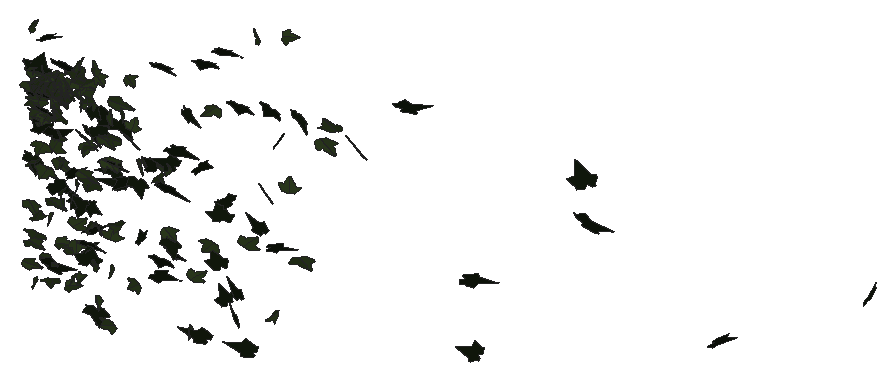
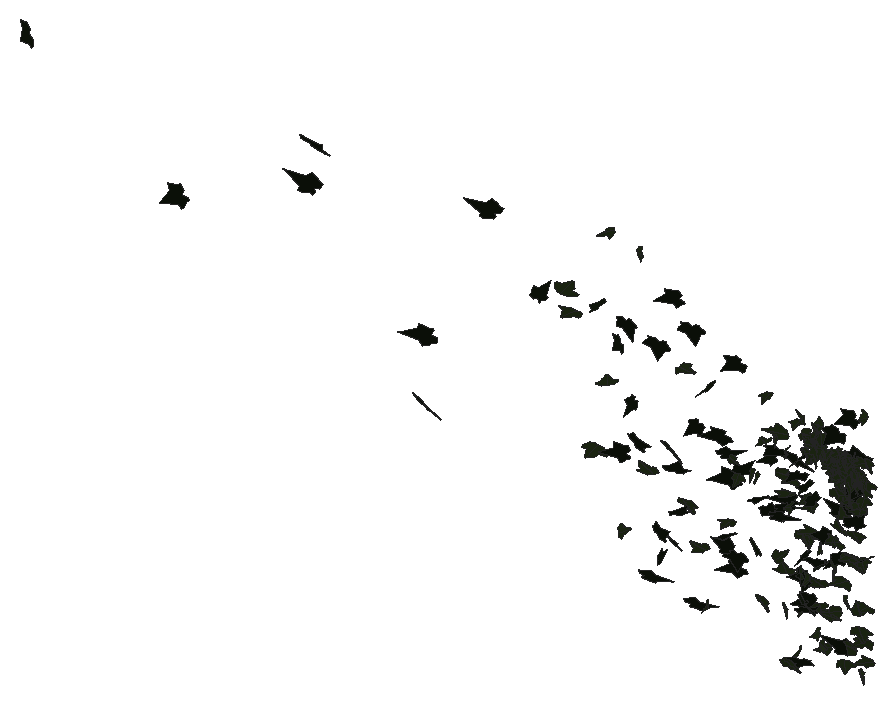
# SketchUp Ruby script. Lengths in millimetres.
U = 1.mm
M = Sketchup.active_model
def pt(a) = Geom::Point3d.new(a.map { |v| v * U })
def face(e, loops, mat)
  f = e.add_face(loops[0].map { |a| pt(a) })
  loops[1..].each { |l| e.add_face(l.map { |a| pt(a) }).erase! }
  f.material = f.back_material = mat if mat
  f
end
# faces: each face lists its corners as indices into pts; further lists are holes
def faces(e, pts, list, mat = nil) = list.each { |f| face(e, (f[0].is_a?(Array) ? f : [f]).map { |l| l.map { |i| pts[i] } }, mat) }
# xy, xz, yz: faces in a plane at the given z, y or x. An outline is a flat list of corners, or four numbers for a rectangle; further outlines are holes
def ring(l) = l.size == 4 ? [[l[0], l[1]], [l[2], l[1]], [l[2], l[3]], [l[0], l[3]]] : l.each_slice(2).to_a
def flat(e, list, mat, &to3) = list.each { |f| face(e, (f[0].is_a?(Array) ? f : [f]).map { |l| ring(l).map { |u, v| to3.(u, v) } }, mat) }
def xy(e, z, list, mat = nil) = flat(e, list, mat) { |x, y| [x, y, z] }
def xz(e, y, list, mat = nil) = flat(e, list, mat) { |x, z| [x, y, z] }
def yz(e, x, list, mat = nil) = flat(e, list, mat) { |y, z| [x, y, z] }
def lines(e, pts, list) = list.each { |a, b| e.add_line(pt(pts[a]), pt(pts[b])) }
# prism: a flat outline (further loops are holes) pulled along v
def prism(e, loops, v, mat = nil)
  f = face(e, loops, mat); d = Geom::Vector3d.new(v.map { |x| x * U })
  f.pushpull(f.normal.samedirection?(d) ? d.length : -d.length)
end
def box(e, o, s, mat = nil) = prism(e, [[o, [o[0] + s[0], o[1], o[2]], [o[0] + s[0], o[1] + s[1], o[2]], [o[0], o[1] + s[1], o[2]]]], [0, 0, s[2]], mat)
def at(x, y, z, deg = 0) = Geom::Transformation.translation(pt([x, y, z])) * Geom::Transformation.rotation(ORIGIN, Z_AXIS, deg.degrees)
def axes(o, x, y, z) = Geom::Transformation.new([*x, 0, *y, 0, *z, 0, *pt(o).to_a, 1])
def part(name) = M.definitions.add(name)
# library, detail: a bought-in or finely detailed component or shape, given as its bounding box
def library(name, o, s) = part(name).tap { |d| box(d.entities, o, s) }
def detail(e, o, s) = box(e.add_group.entities, o, s)
def put(e, d, t, mat = nil) = e.add_instance(d, t).tap { |i| i.material = mat if mat }
def group(e, t, mat = nil) = e.add_group.tap { |g| g.transformation = t; g.material = mat if mat }.entities
root = M.entities
M.materials.add("efeu1").color = [18, 25, 13]
M.materials.add("efeu2").color = [43, 57, 29]
c1 = part("ivyleaf_10")
p = [[0,12.8,-0.8],[-1.5,51.3,-10.9],[-4.9,51,-11.6],[-13.6,26.5,-7.3],[-13.2,15.9,-4.6],[-21.1,19.3,-7.2],
  [-29.5,16.3,-8.3],[-29.2,8.3,-6.2],[-19.7,-9.8,0.5],[-7.6,-13,4],[1,-12.2,5.8],[-0.4,51.1,-11.1],
  [-1.5,51.1,-10.9],[1,-12.4,5.9],[16.9,-12.4,3.5],[35.1,9.1,-5.1],[35,12.9,-6.1],[20.5,16.4,-4.9],
  [15.8,15,-3.8],[15.3,27.6,-7.1],[12.8,31.3,-7.8]]
faces(c1.entities,p,[[0,1,2,3,4,5,6,7,8,9,10],[11,12,0,13,14,15,16,17,18,19,20]],"efeu2")
c2 = part("ivyleaf_9")
p = [[39.1,54.8,31.7],[34.5,51.8,30.2],[-5.3,25.2,17.3],[-17.9,28.3,20.9],[-21.6,21.7,17],[-20.2,4.3,5.3],
  [-22.9,-0.3,2.5],[-17.1,-4,-0.6],[-2,-2.1,-1.2],[-0.7,-15.4,-10.1],[16.6,-22.3,-16.7],[21.1,-15.1,-12.5],
  [32.7,-10.7,-11],[46.1,-1.8,-6.6],[30.8,11.2,3.8]]
faces(c2.entities,p,[[0,1,2,3,4,5,6,7,8,9,10,11,12,13,14]],"efeu1")
put(root,c1,axes([2112,1020.5,1086.8],[0.90728,-0.38712,-0.39338],[-0.36236,0.37255,-0.59734],[0.98591,0.49317,0.14246]))
put(root,c1,axes([2113.2,1028.1,1008.5],[-0.24913,0.51689,0.45995],[-0.42077,0.41232,-0.52628],[-1.24779,-0.24224,0.08564]))
put(root,c1,axes([2102.4,1029.6,1001.6],[1.26935,0.2079,0.08704],[0.12033,0.08839,-0.69557],[-0.41173,0.66678,0.06506]))
put(root,c1,axes([2093.7,1044.4,513.5],[1.2228,0.0441,0.3558],[0.67624,0.01901,-0.64399],[-0.09096,0.73419,-0.0047]))
put(root,c1,axes([2116.9,1041.1,689.2],[-0.35833,-0.7134,0.01011],[-0.00148,-0.01025,-0.73783],[1.35789,-0.18827,0.00186]))
put(root,c1,axes([2095.1,1025.5,281.6],[0.29815,0.15875,0.68166],[0.75147,0.5567,-0.22039],[-1.09983,0.42341,0.0342]))
put(root,c2,axes([2104.3,1048.7,702.6],[-0.18875,-0.81121,0.04789],[0.00119,-0.04832,-0.81722],[1.54657,-0.09897,0.00647]))
put(root,c1,axes([2113.3,1037.3,935.7],[-0.62489,-0.56416,-0.21139],[0.29535,0.15342,-0.6505],[1.10791,-0.3591,0.05418]))
put(root,c1,axes([2129.6,1039.7,405.6],[-1.32292,-0.22351,0.24764],[-0.44428,-0.08297,-0.73012],[0.45354,-0.73322,0.00713]))
put(root,c1,axes([2111.3,1037.6,979.9],[1.25171,-0.35349,0.12885],[0.21425,-0.06272,-0.74666],[0.68326,0.66725,-0.00192]))
put(root,c1,axes([2106.2,1037,367.9],[-0.98081,-0.23976,-0.514],[0.89991,0.20192,-0.56826],[0.59614,-0.69929,0.01215]))
put(root,c1,axes([2128.9,1009,1250.8],[0.20732,-0.22987,0.78589],[-0.41846,0.75549,0.25145],[-1.50115,-0.24235,0.03844]))
put(root,c1,axes([2131.7,1032.7,1028.2],[0.0382,-0.70948,-0.05814],[-0.01252,0.05797,-0.70974],[1.35474,0.02054,-0.00492]))
put(root,c1,axes([2126.5,1041.1,1002.5],[0.6917,-0.52586,0.27284],[0.29553,-0.22435,-0.63923],[1.08809,0.39522,0.00017]))
put(root,c1,axes([2128.9,1037.5,988.7],[-0.2142,0.67192,0.11822],[-0.05171,0.11531,-0.68123],[-1.2974,-0.11553,0.00764]))
put(root,c1,axes([2148.1,1028.3,905.3],[-0.9668,-0.28055,0.40562],[-0.64451,-0.22491,-0.57967],[0.68238,-0.60991,0.02718]))
put(root,c1,axes([2134.8,1023.6,224.3],[0.3777,-0.71041,-0.10598],[-0.03292,0.10519,-0.73752],[1.36661,0.19888,0.01153]))
put(root,c1,axes([2137.3,1034.1,1004.6],[0.21231,-0.69891,0.03845],[-0.0287,-0.04133,-0.70744],[1.33187,0.11052,-0.02137]))
put(root,c1,axes([2128.4,1037.3,885.3],[0.85929,0.51129,0.06191],[0.08647,0.04246,-0.68208],[-0.97638,0.45374,-0.00592]))
put(root,c1,axes([2143.1,1029.3,1016.8],[-1.28026,-0.16554,0.06589],[-0.11694,-0.02603,-0.69267],[0.31829,-0.6754,0.01055]))
put(root,c1,axes([2134.3,1034.1,1023.8],[0.87913,-0.53007,0.10724],[0.20821,-0.04653,-0.70122],[1.00799,0.47192,0.05131]))
put(root,c1,axes([2136.4,1033.9,473.7],[-0.55777,-0.67097,-0.04109],[-0.03086,-0.03776,0.73218],[-1.279,0.29352,0.00026]))
put(root,c2,axes([2147.2,1050.1,827.2],[0.68325,0.22956,0.7152],[-1.28524,-0.24845,0.41872],[0.62596,-0.7607,0.07907]))
put(root,c1,axes([2162.3,1029.7,961.1],[0.32073,0.04351,-0.68613],[-1.29818,-0.07779,-0.17247],[-0.16369,0.70223,0.02341]))
put(root,c1,axes([2126.2,1011.6,1071.8],[0.43174,0.20136,0.66661],[0.52908,0.61661,-0.28086],[-1.21511,0.34003,0.11456]))
put(root,c1,axes([2161.5,1040.1,670.2],[0.88145,-0.15238,-0.52506],[-0.88555,0.25145,-0.4834],[0.54633,0.65342,0.06358]))
put(root,c1,axes([2150.1,1034.5,1029.5],[-0.16422,-0.70447,0.00916],[0.00312,-0.00943,-0.70973],[1.34086,-0.08626,0.00278]))
put(root,c2,axes([2140,1021.6,982.3],[1.3003,0.38247,-0.13387],[-0.21891,-0.06859,-0.78298],[-0.7395,0.69282,-0.00361]))
put(root,c2,axes([2151.4,1016.1,1086.7],[-1.35869,0.19389,0.41929],[0.77286,-0.10451,0.73974],[0.4191,0.8213,-0.00485]))
put(root,c1,axes([2156.9,1032.4,985.3],[0.34982,-0.67422,-0.05252],[-0.01971,0.05161,-0.69881],[1.28691,0.18406,0.00357]))
put(root,c1,axes([2157.8,1039.1,1023.9],[0.26832,-0.67536,0.11177],[0.01691,-0.1123,-0.68978],[1.30273,0.14056,-0.01407]))
put(root,c1,axes([2159.8,1034.4,1037.8],[-0.66542,-0.61331,-0.04929],[0.05578,0.04003,-0.70594],[1.16968,-0.35082,0.00562]))
put(root,c1,axes([2160,1027.2,778.9],[1.34867,0.13646,-0.15114],[-0.28116,-0.03209,-0.72164],[-0.26672,0.72386,-0.0035]))
put(root,c1,axes([2163.4,1042.1,1007.6],[-0.57237,-0.62446,-0.04999],[0.14646,0.01821,-0.69039],[1.18325,-0.30432,0.06127]))
put(root,c1,axes([2168.6,1039.5,984.6],[-0.46205,-0.61321,-0.22742],[0.12931,0.21763,-0.65932],[1.238,-0.25159,-0.01601]))
put(root,c1,axes([2173.5,1018.5,1087.6],[-0.55871,0.63899,0.22033],[-0.29411,0.1704,-0.70009],[-1.25232,-0.3251,0.06612]))
put(root,c1,axes([2173.2,1033.7,683.7],[1.48548,0.02182,-0.19434],[-0.36955,-0.00855,-0.78082],[-0.04422,0.8043,-0.00303]))
put(root,c1,axes([2173.9,1038,1031.3],[0.47163,-0.65475,-0.05712],[0.02276,0.06553,-0.69924],[1.25065,0.24572,0.03427]))
put(root,c1,axes([2174,1031.1,902.8],[1.00718,0.40547,-0.18058],[-0.25511,-0.12189,-0.66652],[-0.80532,0.54572,-0.0147]))
put(root,c1,axes([2179,1031.2,907.1],[0.41562,-0.68765,0.04104],[0.00973,-0.04144,-0.72145],[1.31102,0.21831,-0.00766]))
put(root,c1,axes([2185.7,1022.9,1017.3],[-0.95033,0.43351,0.23528],[-0.40033,0.11567,-0.65954],[-0.84909,-0.53973,0.04763]))
put(root,c2,axes([2168.7,1018,932.7],[1.41397,-0.01466,-0.22358],[-0.42548,0.0034,-0.74309],[0.02858,0.77585,-0.00097]))
put(root,c1,axes([2158,1036.2,675.7],[0.57865,0.05001,0.64634],[1.1375,0.25487,-0.30087],[-0.47786,0.66726,0.06648]))
put(root,c1,axes([2193.1,1026.4,1044.9],[0.85146,-0.34329,-0.46306],[-0.44929,0.42563,-0.54363],[1.00083,0.48313,0.1499]))
put(root,c1,axes([2161.9,1039.8,318.6],[-0.01053,0.02222,-0.80273],[1.23386,-0.47358,-0.01758],[-0.90188,-0.64817,-0.01467]))
put(root,c1,axes([2193.9,1023.2,1068.9],[-0.32616,-0.68086,-0.13484],[0.10236,0.12544,-0.70178],[1.317,-0.17836,0.02115]))
put(root,c1,axes([2199.3,1030.1,912.1],[-0.95954,-0.47222,0.0787],[-0.11929,-0.0482,-0.69074],[0.90329,-0.508,-0.00762]))
put(root,c1,axes([2198.4,1027.6,1069],[-1.32419,0.14245,0.06295],[-0.11397,0.02136,-0.71015],[-0.27361,-0.69828,-0.00888]))
put(root,c1,axes([2196.6,1032.6,1044.4],[0.21055,-0.69926,0.00613],[0.00176,-0.00606,-0.70796],[1.33088,0.11064,-0.00003]))
put(root,c1,axes([2206.2,1031.4,1070.5],[0.47919,0.2857,-0.60647],[-0.84856,-0.41243,-0.37939],[-0.95282,0.51099,0.03288]))
put(root,c2,axes([2181.7,1008.1,1228.6],[0.83231,0.3907,0.59865],[0.76072,0.44819,-0.5845],[-1.12799,0.59055,0.04754]))
put(root,c1,axes([2202.3,1035,246.5],[-0.89756,-0.55993,0.02203],[-0.00643,-0.02595,-0.73194],[1.06647,-0.47141,0.01412]))
put(root,c1,axes([2194.2,1038.9,501.9],[0.54311,-0.58316,0.33017],[0.2819,-0.2951,-0.64923],[1.24387,0.32151,0.00297]))
put(root,c1,axes([2206.1,1023.9,1078.3],[-0.79031,-0.599,-0.06841],[0.05009,0.06498,-0.72869],[1.14633,-0.4158,-0.01532]))
put(root,c1,axes([2207,1037.3,975.1],[0.22655,0.69325,0.00408],[-0.00255,0.00437,-0.70339],[-1.31942,0.11903,0.00206]))
put(root,c1,axes([2216.3,1030.6,1068.9],[0.70918,-0.59763,-0.12575],[-0.13344,0.10447,-0.70427],[1.15464,0.37914,-0.00415]))
put(root,c1,axes([2187.9,1039.6,1021.1],[0.02204,-0.07304,0.69553],[1.289,0.17457,0.00705],[-0.33177,0.67337,0.07361]))
put(root,c1,axes([2209.9,1034.6,1038],[-1.23402,0.09629,-0.2497],[0.44204,-0.12268,-0.65042],[-0.25305,-0.6839,0.08152]))
put(root,c1,axes([2218.9,1036.3,982],[-0.69589,0.60279,-0.01072],[-0.07592,-0.0367,-0.70301],[-1.1449,-0.36396,0.05313]))
put(root,c1,axes([2207.8,1042.2,779.5],[1.35633,-0.41458,-0.15108],[0.26282,-0.06302,0.82434],[-0.79761,-0.72577,0.01472]))
put(root,c1,axes([2239.7,1020.7,956.9],[-0.55329,0.21104,0.62694],[-1.09349,0.25883,-0.35355],[-0.62394,-0.64076,0.06367]))
put(root,c1,axes([2213.9,1035,981.9],[1.25345,0.19342,-0.16119],[0.231,0.1516,0.67782],[0.41985,-0.66087,0.10831]))
put(root,c1,axes([2213,1029.6,1075.7],[1.18609,-0.34286,0.12479],[0.34236,0.07383,-0.69549],[0.60416,0.63128,0.14912]))
put(root,c1,axes([2205.9,1029.8,570.2],[-0.9974,-0.02971,-0.53153],[1.01009,0.02912,-0.5249],[0.07916,-0.74587,0.00068]))
put(root,c1,axes([2226.3,1031.3,830.7],[-1.34791,0.0057,0.0145],[0.02748,-0.00699,0.70823],[0.01111,0.70835,0.00687]))
put(root,c2,axes([2191.5,1033.1,302],[0.36992,-0.07367,0.84761],[1.48021,-0.33712,-0.20765],[0.6565,0.80161,-0.00942]))
put(root,c1,axes([2244.8,1029.6,920.4],[-1.03647,0.07206,0.44525],[-0.83434,0.07964,-0.54909],[-0.20193,-0.69892,-0.01666]))
put(root,c1,axes([2230.2,1028,1029.2],[0.24637,-0.69706,0.04803],[0.00638,-0.04823,-0.70896],[1.32977,0.12938,-0.0055]))
put(root,c1,axes([2235.4,1027.9,1080.2],[-0.67295,0.50507,0.35484],[-0.45094,0.26655,-0.6155],[-1.08477,-0.42413,0.03573]))
put(root,c1,axes([2230.8,1028.5,1087.4],[0.43683,-0.67108,0.12069],[0.12229,-0.10549,-0.70876],[1.29191,0.2369,0.02628]))
put(root,c1,axes([2217.8,1028.6,1082.7],[0.7132,0.36428,0.49339],[0.63155,0.36583,-0.52213],[-0.98162,0.50003,0.02255]))
put(root,c2,axes([2215.1,1022.9,841.6],[-0.23057,-0.11905,0.76279],[1.46767,-0.05525,0.11386],[0.06962,0.77038,0.12604]))
put(root,c1,axes([2235.2,1034.5,992.7],[-1.25751,0.11765,-0.22453],[0.41788,-0.04762,-0.67108],[-0.24108,-0.69622,0.00796]))
put(root,c1,axes([2237.7,1051,726.6],[-0.01547,-0.07625,0.70936],[0.49261,-0.66139,-0.06813],[1.26532,0.25656,0.03519]))
put(root,c2,axes([2234.6,1011.3,654.6],[0.12684,-0.17459,-0.86218],[-0.3024,0.84804,-0.18401],[1.64668,0.16919,0.03262]))
put(root,c1,axes([2239.1,1025.2,1019.6],[-0.82074,-0.2955,-0.48237],[0.76741,0.26485,-0.52272],[0.75511,-0.59035,0.00694]))
put(root,c1,axes([2248.3,1028.6,1011.3],[-0.6581,0.60475,-0.1129],[0.00283,-0.12869,-0.69388],[-1.17084,-0.34022,0.06178]))
put(root,c1,axes([2224.2,1044,727.5],[0.95157,-0.01298,0.67816],[1.29083,-0.0003,-0.50005],[0.01512,0.84255,0.01028]))
put(root,c1,axes([2250,1036.3,1039.3],[0.00764,0.699,-0.0965],[-0.00528,-0.09649,-0.69901],[-1.34294,0.00436,0.0022]))
put(root,c1,axes([2258.4,1028.6,636.1],[0.15707,-0.74652,-0.09178],[-0.01922,0.09122,-0.75107],[1.43135,0.08315,-0.00001]))
put(root,c1,axes([2265.4,1015.5,578.5],[0.08954,-0.01852,-0.75265],[-0.22033,0.74497,-0.02557],[1.41583,0.1171,0.04362]))
put(root,c1,axes([2260.9,1034.1,1008.4],[0.78453,-0.492,-0.30715],[-0.02716,0.3681,-0.60879],[1.10354,0.35884,0.20338]))
put(root,c2,axes([2247.5,1015.1,1149.4],[1.57467,0.13468,-0.12334],[-0.23309,-0.01528,-0.83826],[-0.25782,0.83639,0.00454]))
put(root,c1,axes([2249.9,1033.7,1029.7],[-1.01332,-0.11728,-0.45636],[0.89131,-0.05584,-0.53203],[0.09881,-0.69902,0.11907]))
put(root,c1,axes([2263.8,1033.3,1009.6],[-0.79761,0.55041,-0.16861],[-0.02268,-0.21681,-0.67814],[-1.09536,-0.3963,0.13682]))
put(root,c1,axes([2267.2,1024.1,1061.9],[1.09385,-0.40155,-0.1105],[-0.1422,0.08585,-0.70059],[0.77978,0.57894,0.02724]))
put(root,c1,axes([2265.8,1034.9,1049.9],[-0.18489,0.68383,-0.15728],[-0.10184,-0.16553,-0.68668],[-1.33156,-0.08229,0.07436]))
put(root,c1,axes([2293.7,1024.9,405],[0.15786,0.10844,0.7082],[-1.34398,-0.10803,0.09925],[0.23028,-0.70481,0.09375]))
put(root,c1,axes([2253.2,1010.6,426.5],[-0.2873,-0.11057,-0.78905],[1.06978,0.55439,-0.18523],[1.07472,-0.58141,-0.02656]))
put(root,c1,axes([2272.7,1027.6,1074.3],[-0.25562,0.69408,0.08027],[-0.02651,0.07906,-0.70696],[-1.32952,-0.13503,-0.00134]))
put(root,c1,axes([2292.7,1031.8,1063.6],[0.08622,-0.71444,-0.00629],[-0.04031,0.00496,-0.71557],[1.35918,0.04547,-0.02082]))
put(root,c1,axes([2297.9,1033.3,1072.3],[0.45945,-0.6636,-0.10336],[0.01678,0.11295,-0.70462],[1.27808,0.23707,0.04641]))
put(root,c1,axes([2295.9,1043.8,289.5],[0.33074,-0.53167,0.51439],[0.2913,-0.49112,-0.55933],[1.37749,0.23152,-0.00523]))
put(root,c1,axes([2305.1,1030.9,1035.5],[0.22875,-0.70701,0.0361],[-0.00472,-0.03704,-0.71711],[1.34733,0.11991,-0.00864]))
put(root,c1,axes([2293.2,1012.6,266.8],[-0.05934,-0.14763,-0.75567],[0.92753,0.58172,-0.13375],[1.13447,-0.48333,0.06983]))
put(root,c1,axes([2317.5,1025.9,1120.5],[-1.30951,-0.1788,0.09769],[-0.18706,-0.01011,-0.71076],[0.33967,-0.69489,-0.0148]))
put(root,c2,axes([2296.8,1014.4,713.7],[0.27346,0.10171,0.75796],[1.05105,0.5197,-0.17443],[-1.00685,0.57014,0.02378]))
put(root,c2,axes([2306.9,1046.3,599.9],[-0.4352,-0.49886,0.64454],[-0.22252,-0.64243,-0.53871],[1.53515,-0.23454,0.10464]))
put(root,c1,axes([2322,1020.1,669.7],[0.05719,-0.21545,-0.73211],[-0.04825,0.73199,-0.21646],[1.45163,0.03282,0.02165]))
put(root,c1,axes([2315.2,1029.6,436.1],[0.78407,0.62153,-0.13019],[-0.15558,-0.10199,-0.74558],[-1.19852,0.41984,0.01161]))
put(root,c1,axes([2325.1,1018,1153.2],[0.19936,-0.48607,0.70488],[-0.35425,0.68022,0.49673],[-1.5906,-0.21242,-0.02228]))
put(root,c1,axes([2329.4,1021.7,1142.8],[0.10108,-0.44146,-0.5868],[0.10664,0.58906,-0.43809],[1.39348,-0.01306,0.07609]))
put(root,c1,axes([2333.5,1028.4,1057.8],[-0.65475,-0.6289,-0.01701],[0.0175,0.01436,-0.71684],[1.19723,-0.34415,0.00117]))
put(root,c1,axes([2316.3,1022.7,515.5],[1.00294,0.21784,-0.49866],[0.85979,0.21184,0.56996],[0.57736,-0.69389,0.01746]))
put(root,c1,axes([2329.4,1023.5,1083.7],[1.17347,0.36267,0.07531],[0.09536,0.06324,-0.71474],[-0.69847,0.61793,0.02895]))
put(root,c2,axes([2338.8,1031.3,611.6],[-1.12044,-0.4398,-0.24676],[0.37003,0.15205,-0.73483],[0.88558,-0.61997,-0.00517]))
put(root,c1,axes([2341.7,1036.2,1091.5],[0.69347,-0.6172,-0.02093],[-0.0181,0.01869,-0.71672],[1.17518,0.36449,0.00131]))
put(root,c1,axes([2339.5,1028.8,1017.6],[0.49597,-0.65105,0.14646],[0.29024,-0.09497,-0.69351],[1.23645,0.28345,0.10404]))
put(root,c1,axes([2340.8,1008,310.1],[-0.0049,-0.06448,-0.77656],[0.37231,0.75164,-0.06306],[1.43554,-0.19516,0.0137]))
put(root,c1,axes([2346.4,1026.3,1145],[0.73669,-0.60528,-0.07917],[-0.0687,0.07089,-0.71843],[1.15975,0.38868,0.00774]))
put(root,c1,axes([2345.4,1042,835.5],[0.68721,0.61203,-0.161],[-0.1893,-0.12818,-0.71032],[-1.18947,0.37399,0.02003]))
put(root,c2,axes([2324.5,1052.7,863.7],[0.54985,-0.58933,0.41729],[0.51026,-0.32978,-0.65137],[1.27609,0.38581,0.08065]))
put(root,c1,axes([2350.3,1025,1017.6],[0.20352,0.24991,0.66756],[-0.09403,0.676,-0.24515],[-1.35334,-0.00939,0.11742]))
put(root,c1,axes([2339.5,1028.6,1086.6],[-0.68248,-0.33781,0.53088],[0.73334,0.36519,0.49265],[-0.9468,0.52636,-0.00109]))
put(root,c1,axes([2336.8,1034.4,723.3],[0.73338,0.09768,0.6969],[1.21165,0.29015,-0.39269],[-0.57065,0.7416,0.06185]))
put(root,c1,axes([2366.6,1049,696.2],[0.26789,-0.72035,0.1083],[0.0351,-0.10674,-0.73397],[1.38593,0.14194,-0.00235]))
put(root,c2,axes([2341.8,1033.3,444.2],[1.30058,0.09355,0.33582],[0.62255,0.08341,-0.68888],[-0.22938,0.75684,0.03441]))
put(root,c1,axes([2374.2,1022.8,516.5],[0.11305,-0.09073,0.83556],[-0.53515,0.78724,0.10547],[-1.50742,-0.28628,0.02522]))
put(root,c1,axes([2386,1028.5,701.9],[-1.50166,-0.18181,0.3115],[-0.57584,-0.07418,-0.80968],[0.37363,-0.84503,0.00406]))
put(root,c2,axes([2385.8,1032.7,444.3],[-0.5577,0.70506,-0.12806],[0.08351,-0.12045,-0.76351],[-1.36126,-0.29624,0.00563]))
put(root,c1,axes([2382.7,1035.4,1110.6],[0.28204,0.35248,-0.60973],[-0.82226,-0.44657,-0.36316],[-1.05855,0.4408,0.11964]))
put(root,c1,axes([2365.7,1024.7,853.1],[-0.32795,-0.34701,-0.67658],[0.62341,0.59219,-0.38715],[1.30599,-0.36982,0.01491]))
put(root,c1,axes([2354.3,1028.1,1065.6],[0.71885,-0.25759,-0.56297],[0.88683,-0.31593,0.45718],[-0.77581,-0.59982,0.00097]))
put(root,c1,axes([2389.3,1025.4,1033.8],[0.75051,-0.29593,-0.5332],[-0.64684,0.42056,-0.48477],[0.96365,0.51277,0.08987]))
put(root,c2,axes([2381.3,1020.9,386.8],[-1.20063,-0.329,0.56453],[0.95259,0.26111,0.71148],[-0.79938,0.80529,-0.00005]))
put(root,c2,axes([2378,1020.4,519.1],[0.50642,0.67068,0.27237],[0.20192,0.25093,-0.72151],[-1.36281,0.2864,-0.00569]))
put(root,c2,axes([2361.9,1044.4,904.1],[0.53107,-0.71441,0.17284],[0.16453,-0.1517,-0.76657],[1.38919,0.29108,0.02471]))
put(root,c2,axes([2385.3,1018.3,616.3],[0.48926,-0.26263,-0.66624],[-0.60028,0.59399,-0.35585],[1.22363,0.3964,0.09182]))
put(root,c1,axes([2403.2,1025.6,1158.6],[0.92762,-0.3415,0.42417],[-0.64962,0.25196,0.59507],[-0.80754,-0.59498,0.00854]))
put(root,c1,axes([2396.6,1045.6,234.2],[-0.08807,0.70809,-0.26757],[0.03238,-0.26702,-0.7096],[-1.44028,-0.0493,0.00041]))
put(root,c2,axes([2390.6,1020.3,1010.3],[0.60025,-0.46545,-0.56839],[-0.34135,0.55105,-0.55077],[1.35587,0.34479,0.11296]))
put(root,c1,axes([2403.6,1031.9,372.2],[-0.54296,0.625,0.35081],[0.23411,-0.32929,0.68667],[1.34383,0.30989,0.02212]))
put(root,c2,axes([2399.2,1039.5,191.7],[-0.86409,-0.49592,-0.38339],[0.50177,0.2784,-0.67234],[1.08234,-0.52499,0.00562]))
put(root,c2,axes([2393.3,1020.5,517.6],[0.44378,0.16249,0.71968],[0.92638,0.53333,-0.27812],[-1.05524,0.53654,0.05851]))
put(root,c1,axes([2416.1,1030.5,522.7],[-0.93547,0.57496,0.06376],[0.04011,-0.06582,0.75595],[1.10023,0.49126,0.02666]))
put(root,c2,axes([2448.8,1030.3,993.1],[-0.66546,-0.06598,-0.81149],[-1.52345,-0.13349,0.35575],[-0.28309,0.87347,-0.00692]))
put(root,c1,axes([2414.8,1026,1144],[0.3698,0.65773,0.24751],[0.06282,0.24797,-0.68487],[-1.33602,0.19372,0.03631]))
put(root,c2,axes([2409.1,1027.8,933.6],[-0.00786,-0.36844,-0.6807],[0.10852,0.67872,-0.36771],[1.46911,-0.05211,0.02352]))
put(root,c1,axes([2465.7,1030.5,158.9],[0.86831,-0.13028,-0.61839],[-1.09762,0.22604,-0.47311],[0.49181,0.73448,0.03592]))
put(root,c1,axes([2446.1,1025.9,786.7],[0.07934,0.2036,-0.79346],[0.39127,0.76646,0.20747],[1.50914,-0.20942,-0.01208]))
put(root,c1,axes([2434.6,1030.4,901.3],[0.9859,0.05372,0.52739],[0.9748,0.13943,-0.5173],[-0.26017,0.72598,0.06032]))
put(root,c2,axes([2482.5,1051.6,778.7],[-0.64632,-0.20304,0.67929],[-1.12733,-0.33266,-0.39556],[0.74153,-0.68271,-0.00928]))
put(root,c1,axes([2490.4,1033.5,912.4],[0.12063,0.08455,-0.74239],[-1.42135,0.03041,-0.0603],[0.04435,0.74447,0.08678]))
put(root,c1,axes([2471.5,1035.9,379.6],[0.36906,-0.66201,-0.33805],[-0.18316,0.32407,-0.68983],[1.4028,0.21648,-0.00113]))
put(root,c2,axes([2446.4,1019.8,815.3],[1.21797,-0.05397,0.40628],[0.7765,0.01244,-0.64102],[0.07398,0.75793,0.03945]))
put(root,c1,axes([2480.4,1016.2,992.1],[-0.12879,0.56097,-0.48379],[-0.1073,0.48049,0.56504],[1.40574,0.08807,-0.00119]))
put(root,c2,axes([2506.6,1046,736.7],[-0.79041,-0.05704,0.67023],[-1.26024,-0.10386,-0.41915],[0.22514,-0.7816,0.00678]))
put(root,c1,axes([2472.9,1026.9,518.7],[1.25741,0.34913,-0.17887],[0.29306,0.09142,0.74721],[0.68667,-0.67834,0.00864]))
put(root,c1,axes([2465,1017.8,827],[0.9484,0.52107,0.39712],[0.53339,0.28144,-0.72096],[-1.12702,0.57168,-0.00703]))
put(root,c1,axes([2501.2,1039.8,566.8],[-0.29779,-0.28352,-0.80973],[-0.70012,-0.72142,0.32368],[-1.47511,0.39964,0.00984]))
put(root,c1,axes([2485.7,1025,1070],[0.24913,-0.02135,0.88207],[1.48658,0.41754,-0.10581],[-0.781,0.78794,0.07997]))
put(root,c2,axes([2534.5,1045,761.5],[0.09778,0.35987,-0.70654],[-0.18739,-0.69964,-0.36352],[-1.49738,0.11105,-0.00064]))
put(root,c2,axes([2511.5,1024,995.8],[-0.46524,-0.32961,-0.64417],[0.84439,0.46886,-0.40827],[1.08792,-0.50486,0.04141]))
put(root,c1,axes([2532.5,1015.3,1041],[0.61846,-0.53129,-0.4965],[-0.11135,0.52295,-0.59789],[1.37947,0.28041,0.17433]))
put(root,c2,axes([2525.9,1027.4,957],[1.15802,-0.46082,0.01006],[0.0155,-0.00592,-0.76327],[0.8771,0.60851,0.0002]))
put(root,c1,axes([2560.8,1014.7,1194.4],[0.30486,0.65025,0.34878],[-0.02412,0.35927,-0.66399],[-1.40412,0.13501,0.08713]))
put(root,c1,axes([2586.4,1025.1,367.2],[1.00021,-0.45018,-0.41172],[-0.56426,0.28648,-0.69167],[1.01474,0.60303,0.02122]))
put(root,c1,axes([2575.7,1016.3,998.9],[0.6371,0.52048,-0.44431],[0.27371,0.43007,0.61215],[1.27335,-0.35286,0.09072]))
put(root,c2,axes([2585,1036.7,778.7],[-0.30704,-0.73886,-0.15481],[0.07877,0.14941,-0.75622],[1.43457,-0.16634,0.00839]))
put(root,c1,axes([2597.3,1028.9,858.9],[-0.43111,0.70891,-0.17425],[0.09552,-0.1669,-0.74422],[-1.38607,-0.23199,0.00291]))
put(root,c2,axes([2618.6,1013.8,563.3],[-0.00282,0.44784,0.67347],[-0.00385,0.67347,-0.44785],[-1.53927,-0.0025,-0.00012]))
put(root,c1,axes([2619.8,1027.9,868.8],[-0.7142,0.59932,0.29821],[-0.31707,0.2475,-0.70706],[-1.23395,-0.41048,0.00908]))
put(root,c2,axes([2663.8,1041.9,859.6],[0.32099,0.16757,0.74554],[-1.2857,-0.32413,0.22568],[0.67969,-0.69225,0.0748]))
put(root,c1,axes([2683.2,1032,832.5],[-0.40155,-0.64049,-0.40511],[0.32642,0.36925,-0.67312],[1.40492,-0.26886,0.04061]))
put(root,c2,axes([2695.1,1025.7,507.8],[1.05616,0.30479,-0.44667],[-0.75575,-0.20476,-0.63306],[-0.69858,0.68231,0.00955]))
put(root,c2,axes([2681.9,1027.3,1286],[1.40183,0.16562,0.11181],[0.19745,0.048,-0.75458],[-0.32503,0.74345,0.02381]))
put(root,c1,axes([2727.4,1023.8,888],[0.52049,-0.23363,-0.69617],[-0.97722,0.47024,-0.35952],[0.99911,0.58165,0.01103]))
put(root,c2,axes([2691.8,1013.1,449.5],[0.25295,0.17433,-0.78554],[0.38129,0.76394,0.20343],[1.48319,-0.22612,0.08167]))
put(root,c2,axes([2745,1037.2,898.8],[-0.27692,-0.0176,0.81186],[-1.45121,-0.28071,-0.14274],[0.53155,-0.77556,0.03324]))
put(root,c1,axes([2724.6,1026.4,630.7],[0.65805,0.59788,0.35399],[0.31208,0.31401,-0.69053],[-1.28502,0.38243,0.01357]))
put(root,c2,axes([2727.2,1043.6,582.6],[-0.26565,-0.76496,-0.11045],[0.05884,0.10662,-0.77751],[1.4698,-0.14253,0.01116]))
put(root,c2,axes([2706.1,1021.8,807.9],[1.57425,-0.12645,0.37067],[0.69248,-0.07239,-0.83663],[0.27579,0.90352,-0.01516]))
put(root,c2,axes([2711.2,1052.9,536.9],[0.47555,-0.3492,0.65781],[0.75822,-0.52355,-0.42926],[1.19756,0.47015,0.01057]))
put(root,c2,axes([2751.6,1030.4,971.3],[0.16448,0.11215,-0.81339],[0.84921,0.68017,0.14119],[1.31182,-0.45437,0.01059]))
put(root,c1,axes([2817.9,1043.6,264.2],[-0.02347,0.55524,-0.56896],[-0.02246,-0.56909,-0.55511],[-1.51284,-0.00016,0.01707]))
put(root,c2,axes([2813.6,1021.1,1146.2],[0.92878,-0.52714,-0.46174],[-0.43636,0.4116,-0.71222],[1.26031,0.53098,0.09369]))
put(root,c2,axes([2884.1,1039,247],[-0.4647,0.06187,0.76441],[-1.44007,0.11133,-0.2507],[-0.23791,-0.7947,0.02439]))
put(root,c1,axes([2840.3,1032.8,482.2],[0.82732,0.27046,-0.61403],[0.9745,0.33909,0.51185],[0.82522,-0.67158,0.01115]))
put(root,c2,axes([2886.7,1037.8,1364],[0.81438,0.52522,-0.40944],[-0.59557,-0.27103,-0.6747],[-1.11881,0.52658,0.06112]))
put(root,c2,axes([2887.2,1005.7,956.8],[-0.1535,0.15868,-0.8708],[-0.5889,0.81418,0.17702],[1.57831,0.31922,-0.01864]))
put(root,c1,axes([2918.9,1031.6,643.9],[1.42024,-0.17636,-0.26112],[-0.47883,0.07067,-0.76673],[0.36107,0.78744,0.01033]))
put(root,c1,axes([2927.7,1040.7,1188.4],[0.67169,0.39946,-0.61544],[-0.87426,-0.41223,-0.53098],[-1.08885,0.5774,0.04668]))
put(root,c2,axes([2964.9,1025.4,578.1],[-1.12127,-0.49016,0.28574],[0.41682,0.18352,0.76639],[-0.99611,0.62854,-0.00095]))
put(root,c2,axes([2965,1040.7,759.8],[-1.37975,-0.23257,0.3128],[0.59164,0.05351,0.76027],[-0.44753,0.78775,0.0407]))
put(root,c2,axes([3005.6,1033.1,844.8],[-0.88057,0.66311,0.16397],[-0.18031,0.13383,-0.80857],[-1.28748,-0.47228,0.00109]))
put(root,c2,axes([3006.3,1012.2,454.2],[-1.23756,0.31147,-0.4384],[-0.79516,0.14052,0.71954],[0.64442,0.77154,0.04593]))
put(root,c2,axes([2963.8,1020.3,1444.9],[1.20357,0.17677,0.4577],[0.81207,0.17049,-0.65539],[-0.46101,0.7618,0.04047]))
put(root,c2,axes([3040.2,1034,474.9],[0.13635,-0.16404,0.80507],[-0.5402,0.75343,0.17878],[-1.46743,-0.2926,0.00899]))
put(root,c2,axes([3037.7,1031.9,370],[0.03792,-0.60547,0.55825],[0.13122,0.55768,0.60239],[-1.56188,0.03216,0.06416]))
put(root,c2,axes([3039.7,1035.7,1246.9],[1.21638,0.27311,-0.45217],[-0.77592,-0.1963,-0.69482],[-0.6393,0.75789,-0.01703]))
put(root,c2,axes([3102.6,1026.9,278.4],[-0.72678,0.07115,0.73811],[-1.38758,0.11553,-0.38833],[-0.25762,-0.82298,0.0093]))
put(root,c1,axes([3084.6,1023.8,705],[1.25769,0.15914,-0.47947],[0.88969,0.10672,0.67971],[0.36457,-0.80945,-0.00465]))
put(root,c1,axes([3148.3,1009.3,1563.9],[-0.05756,0.09779,-0.81771],[-0.56763,0.76141,0.10209],[1.46096,0.29969,0.00745]))
put(root,c2,axes([3161.7,1013.5,791.1],[-0.09853,0.06678,0.83715],[-0.82922,0.71489,-0.08397],[-1.36639,-0.43866,-0.00941]))
put(root,c2,axes([3184,1036.3,1281],[0.8529,0.09059,-0.71612],[-1.34224,-0.12461,-0.45711],[-0.29265,0.83554,0.00947]))
put(root,c2,axes([3165,1018,957.1],[1.23918,-0.29975,-0.51463],[-0.8763,0.23028,-0.71666],[0.71894,0.79734,0.01351]))
put(root,c1,axes([3190,1060.9,440.6],[-0.0992,0.12562,-0.83945],[-0.51735,-0.79921,-0.10272],[-1.53035,0.26204,0.08914]))
put(root,c2,axes([3205.8,1018.6,734.2],[0.89598,0.18764,0.67897],[1.15486,0.30675,-0.50551],[-0.68092,0.76716,0.03606]))
put(root,c2,axes([3232.3,1012.6,1167.5],[0.20044,0.39282,0.75518],[0.42873,0.72094,-0.40642],[-1.56231,0.24824,-0.01465]))
put(root,c1,axes([3265.6,1019.2,1610.9],[0.08489,-0.28403,-0.78881],[0.89484,0.66249,-0.21196],[1.32109,-0.43048,0.19426]))
put(root,c1,axes([3278.1,1023.6,994.5],[0.97843,0.66701,-0.19705],[0.189,0.17214,0.84174],[1.31012,-0.52297,0.02573]))
put(root,c2,axes([3309.9,1035.2,1298],[0.34274,-0.80195,0.27016],[0.138,-0.26057,-0.82182],[1.60462,0.1937,0.01298]))
put(root,c1,axes([3324.6,1033.5,722.1],[-1.37393,-0.43332,-0.42296],[0.71258,0.19783,-0.84172],[0.90572,-0.81296,0.02062]))
put(root,c1,axes([3426.2,1030,1233.9],[1.13784,0.39541,0.50622],[0.80176,0.28069,-0.71679],[-0.92288,0.73137,0.00141]))
put(root,c1,axes([3471.6,1031.2,1303.3],[-1.37577,-0.25905,-0.43576],[-0.77553,-0.15457,0.76785],[-0.57396,0.82978,0.007]))
put(root,c2,axes([3576.8,1042.5,1246.3],[0.78079,-0.78844,0.32455],[-0.23696,0.30091,0.88839],[-1.60533,-0.42789,0.02672]))
put(root,c2,axes([3794.5,1024.1,1504.1],[0.34106,-0.12521,0.94889],[1.80951,0.13429,-0.16184],[-0.20945,0.95628,0.14697]))
put(root,c2,axes([4126.6,1024.3,627.2],[-1.00843,0.61283,0.52621],[-0.63431,0.40739,-0.81004],[-1.40035,-0.62585,-0.01202]))
put(root,c2,axes([4078.7,1029.3,912.2],[0.50181,0.41927,-0.86319],[0.46579,0.83619,0.48091],[1.76596,-0.33969,0.11843]))
put(root,c2,axes([4618.7,1022.5,1491.2],[-1.90032,0.26562,-0.29722],[-0.54656,0.07659,1.03321],[0.52613,1.03897,-0.00018]))
put(root,c2,axes([4604.2,1031,1323.1],[0.5684,-0.2459,1.00252],[1.54644,-0.58764,-0.3862],[1.2116,0.8654,0.02262]))
put(root,c2,axes([5215.6,1005.1,1064.9],[0.80534,0.56634,0.87028],[1.00431,0.69207,-0.70694],[-1.70192,0.67638,-0.00536]))
put(root,c2,axes([5901.3,1007.5,1476.8],[0.30186,0.38807,1.13311],[0.52512,1.10042,-0.4155],[-2.2182,0.31332,0.05584]))
